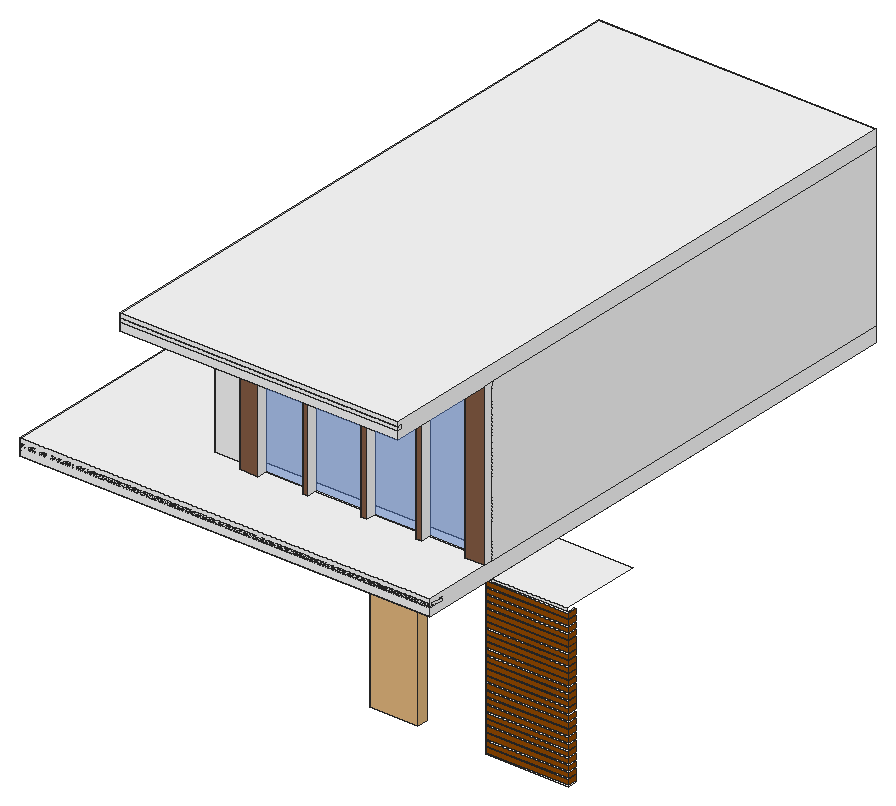
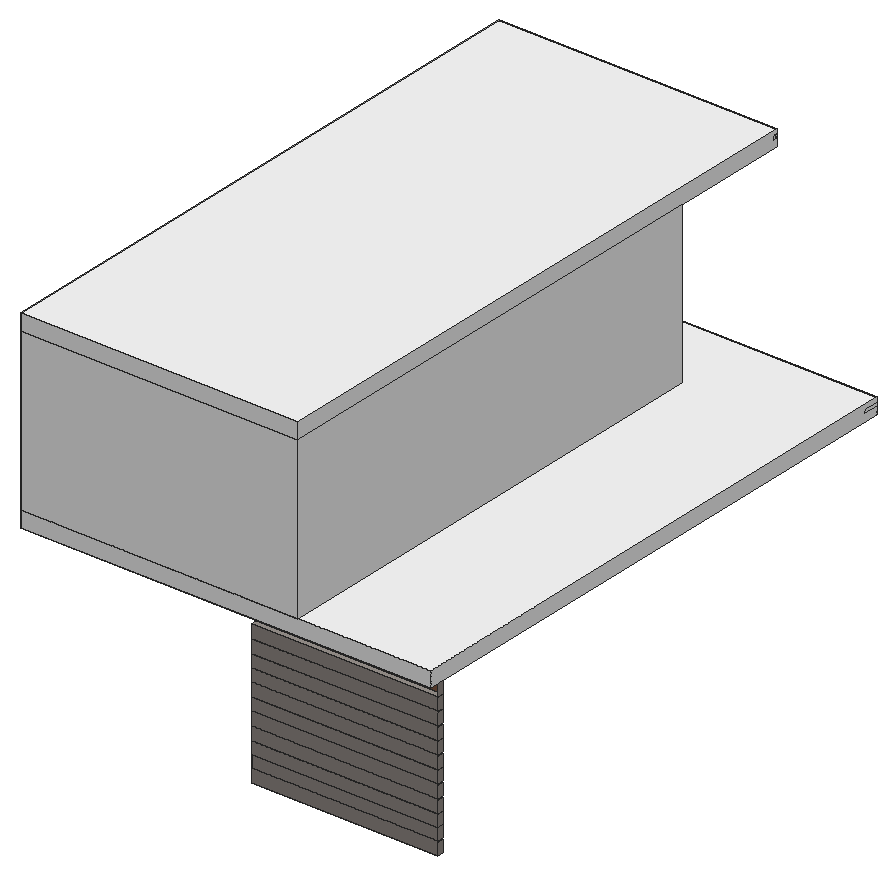
# SketchUp Ruby script. Lengths in inches.
U = 1.inch
M = Sketchup.active_model
def pt(a) = Geom::Point3d.new(a.map { |v| v * U })
def face(e, loops, mat)
  f = e.add_face(loops[0].map { |a| pt(a) })
  loops[1..].each { |l| e.add_face(l.map { |a| pt(a) }).erase! }
  f.material = f.back_material = mat if mat
  f
end
# faces: each face lists its corners as indices into pts; further lists are holes
def faces(e, pts, list, mat = nil) = list.each { |f| face(e, (f[0].is_a?(Array) ? f : [f]).map { |l| l.map { |i| pts[i] } }, mat) }
# xy, xz, yz: faces in a plane at the given z, y or x. An outline is a flat list of corners, or four numbers for a rectangle; further outlines are holes
def ring(l) = l.size == 4 ? [[l[0], l[1]], [l[2], l[1]], [l[2], l[3]], [l[0], l[3]]] : l.each_slice(2).to_a
def flat(e, list, mat, &to3) = list.each { |f| face(e, (f[0].is_a?(Array) ? f : [f]).map { |l| ring(l).map { |u, v| to3.(u, v) } }, mat) }
def xy(e, z, list, mat = nil) = flat(e, list, mat) { |x, y| [x, y, z] }
def xz(e, y, list, mat = nil) = flat(e, list, mat) { |x, z| [x, y, z] }
def yz(e, x, list, mat = nil) = flat(e, list, mat) { |y, z| [x, y, z] }
def lines(e, pts, list) = list.each { |a, b| e.add_line(pt(pts[a]), pt(pts[b])) }
# prism: a flat outline (further loops are holes) pulled along v
def prism(e, loops, v, mat = nil)
  f = face(e, loops, mat); d = Geom::Vector3d.new(v.map { |x| x * U })
  f.pushpull(f.normal.samedirection?(d) ? d.length : -d.length)
end
def box(e, o, s, mat = nil) = prism(e, [[o, [o[0] + s[0], o[1], o[2]], [o[0] + s[0], o[1] + s[1], o[2]], [o[0], o[1] + s[1], o[2]]]], [0, 0, s[2]], mat)
def at(x, y, z, deg = 0) = Geom::Transformation.translation(pt([x, y, z])) * Geom::Transformation.rotation(ORIGIN, Z_AXIS, deg.degrees)
def axes(o, x, y, z) = Geom::Transformation.new([*x, 0, *y, 0, *z, 0, *pt(o).to_a, 1])
def part(name) = M.definitions.add(name)
# library, detail: a bought-in or finely detailed component or shape, given as its bounding box
def library(name, o, s) = part(name).tap { |d| box(d.entities, o, s) }
def detail(e, o, s) = box(e.add_group.entities, o, s)
def put(e, d, t, mat = nil) = e.add_instance(d, t).tap { |i| i.material = mat if mat }
def group(e, t, mat = nil) = e.add_group.tap { |g| g.transformation = t; g.material = mat if mat }.entities
root = M.entities
M.materials.add("[Color C07]").color = [153, 76, 0]
M.materials.add("[Color M00]").color = [255, 255, 255]
M.materials.add("[Granite Tile]").color = [155, 148, 143]
M.materials.add("[Translucent Glass Blue]").color = [100, 149, 237]
M.materials["[Translucent Glass Blue]"].alpha = 0.5
M.materials.add("[Wood Veneer 02]").color = [137, 95, 70]
c1 = library("PINTU 6 YA",[0,-0.6875,0],[35.83,8.07,80.71])
box(root,[257.3125,155.5,390],[307.5,10.6875,2.42],"[Color M00]")
box(root,[356.51,125.125,522],[208.3,2.5625,3.02],"[Color M00]")
xy(root,265.59,[[561.375,211.8125,623.5625,211.8125,623.5625,218.625,622.25,218.625,622.25,213.625,561.375,213.625]],"[Color M00]")
xy(root,266.65,[[561.375,211.8125,561.375,213.625,622.25,213.625,622.25,218.625,623.5625,218.625,623.5625,211.8125]],"[Color M00]")
xy(root,268.5625,[[257.3125,562.2,396.75,566.64]],"[Granite Tile]")
xy(root,270.21,[[561.375,211.8125,623.5625,211.8125,623.5625,218.625,622.25,218.625,622.25,213.625,561.375,213.625]],"[Color M00]")
xy(root,271.27,[[561.375,211.8125,561.375,213.625,622.25,213.625,622.25,218.625,623.5625,218.625,623.5625,211.8125]],"[Color M00]")
xy(root,274.84,[[561.375,211.8125,623.5625,211.8125,623.5625,218.625,622.25,218.625,622.25,213.625,561.375,213.625]],"[Color M00]")
xy(root,276.02,[[561.375,211.8125,561.375,213.625,622.25,213.625,622.25,218.625,623.5625,218.625,623.5625,211.8125]],"[Color M00]")
xy(root,278.5,[[257.3125,562.2,396.75,566.64]],"[Granite Tile]")
xy(root,279.59,[[561.375,211.8125,623.5625,211.8125,623.5625,218.625,622.25,218.625,622.25,213.625,561.375,213.625]],"[Color M00]")
xy(root,280.85,[[561.375,211.8125,561.375,213.625,622.25,213.625,622.25,218.625,623.5625,218.625,623.5625,211.8125]],"[Color M00]")
xy(root,284.41,[[561.375,211.8125,623.5625,211.8125,623.5625,218.625,622.25,218.625,622.25,213.625,561.375,213.625]],"[Color M00]")
xy(root,285.72,[[561.375,211.8125,561.375,213.625,622.25,213.625,622.25,218.625,623.5625,218.625,623.5625,211.8125]],"[Color M00]")
xy(root,287.25,[[257.3125,562.2,396.75,566.64]],"[Granite Tile]")
xy(root,289.29,[[561.375,211.8125,623.5625,211.8125,623.5625,218.625,622.25,218.625,622.25,213.625,561.375,213.625]],"[Color M00]")
xy(root,290.1,[[561.375,211.8125,561.375,213.625,622.25,213.625,622.25,218.625,623.5625,218.625,623.5625,211.8125]],"[Color M00]")
xy(root,293.66,[[561.375,211.8125,623.5625,211.8125,623.5625,218.625,622.25,218.625,622.25,213.625,561.375,213.625]],"[Color M00]")
xy(root,294.97,[[561.375,211.8125,561.375,213.625,622.25,213.625,622.25,218.625,623.5625,218.625,623.5625,211.8125]],"[Color M00]")
xy(root,296.875,[[257.3125,562.2,396.75,566.64]],"[Granite Tile]")
xy(root,298.54,[[561.375,211.8125,623.5625,211.8125,623.5625,218.625,622.25,218.625,622.25,213.625,561.375,213.625]],"[Color M00]")
xy(root,299.91,[[561.375,211.8125,561.375,213.625,622.25,213.625,622.25,218.625,623.5625,218.625,623.5625,211.8125]],"[Color M00]")
xy(root,303.47,[[561.375,211.8125,623.5625,211.8125,623.5625,218.625,622.25,218.625,622.25,213.625,561.375,213.625]],"[Color M00]")
xy(root,304.72,[[561.375,211.8125,561.375,213.625,622.25,213.625,622.25,218.625,623.5625,218.625,623.5625,211.8125]],"[Color M00]")
xy(root,306.5,[[257.3125,562.2,396.75,566.64]],"[Granite Tile]")
xy(root,308.29,[[561.375,211.8125,623.5625,211.8125,623.5625,218.625,622.25,218.625,622.25,213.625,561.375,213.625]],"[Color M00]")
xy(root,309.6,[[561.375,211.8125,561.375,213.625,622.25,213.625,622.25,218.625,623.5625,218.625,623.5625,211.8125]],"[Color M00]")
xy(root,313.16,[[561.375,211.8125,623.5625,211.8125,623.5625,218.625,622.25,218.625,622.25,213.625,561.375,213.625]],"[Color M00]")
xy(root,314.54,[[561.375,211.8125,561.375,213.625,622.25,213.625,622.25,218.625,623.5625,218.625,623.5625,211.8125]],"[Color M00]")
xy(root,316.5625,[[257.3125,562.2,396.75,566.64]],"[Granite Tile]")
xy(root,318.1,[[561.375,211.8125,623.5625,211.8125,623.5625,218.625,622.25,218.625,622.25,213.625,561.375,213.625]],"[Color M00]")
xy(root,319.1,[[561.375,211.8125,561.375,213.625,622.25,213.625,622.25,218.625,623.5625,218.625,623.5625,211.8125]],"[Color M00]")
xy(root,322.66,[[561.375,211.8125,623.5625,211.8125,623.5625,218.625,622.25,218.625,622.25,213.625,561.375,213.625]],"[Color M00]")
xy(root,323.85,[[561.375,211.8125,561.375,213.625,622.25,213.625,622.25,218.625,623.5625,218.625,623.5625,211.8125]],"[Color M00]")
xy(root,326.4375,[[257.3125,562.2,396.75,566.64]],"[Granite Tile]")
xy(root,327.41,[[561.375,211.8125,623.5625,211.8125,623.5625,218.625,622.25,218.625,622.25,213.625,561.375,213.625]],"[Color M00]")
xy(root,328.35,[[561.375,211.8125,561.375,213.625,622.25,213.625,622.25,218.625,623.5625,218.625,623.5625,211.8125]],"[Color M00]")
xy(root,331.91,[[561.375,211.8125,623.5625,211.8125,623.5625,218.625,622.25,218.625,622.25,213.625,561.375,213.625]],"[Color M00]")
xy(root,333.1,[[561.375,211.8125,561.375,213.625,622.25,213.625,622.25,218.625,623.5625,218.625,623.5625,211.8125]],"[Color M00]")
xy(root,336.1875,[[257.3125,562.2,396.75,566.64]],"[Granite Tile]")
xy(root,336.66,[[561.375,211.8125,623.5625,211.8125,623.5625,218.625,622.25,218.625,622.25,213.625,561.375,213.625]],"[Color M00]")
xy(root,337.48,[[561.375,211.8125,561.375,213.625,622.25,213.625,622.25,218.625,623.5625,218.625,623.5625,211.8125]],"[Color M00]")
xy(root,341.04,[[561.375,211.8125,623.5625,211.8125,623.5625,218.625,622.25,218.625,622.25,213.625,561.375,213.625]],"[Color M00]")
xy(root,342.04,[[561.375,211.8125,561.375,213.625,622.25,213.625,622.25,218.625,623.5625,218.625,623.5625,211.8125]],"[Color M00]")
xy(root,345.6,[[561.375,211.8125,623.5625,211.8125,623.5625,218.625,622.25,218.625,622.25,213.625,561.375,213.625]],"[Color M00]")
xy(root,345.875,[[257.3125,562.2,396.75,566.64]],"[Granite Tile]")
xy(root,346.54,[[561.375,211.8125,561.375,213.625,622.25,213.625,622.25,218.625,623.5625,218.625,623.5625,211.8125]],"[Color M00]")
xy(root,350.1,[[561.375,211.8125,623.5625,211.8125,623.5625,218.625,622.25,218.625,622.25,213.625,561.375,213.625]],"[Color M00]")
xy(root,350.85,[[561.375,211.8125,561.375,213.625,622.25,213.625,622.25,218.625,623.5625,218.625,623.5625,211.8125]],"[Color M00]")
xy(root,354.41,[[561.375,211.8125,623.5625,211.8125,623.5625,218.625,622.25,218.625,622.25,213.625,561.375,213.625]],"[Color M00]")
xy(root,355.35,[[561.375,211.8125,561.375,213.625,622.25,213.625,622.25,218.625,623.5625,218.625,623.5625,211.8125]],"[Color M00]")
xy(root,355.4375,[[257.3125,562.2,396.75,566.64]],"[Granite Tile]")
xy(root,358.91,[[561.375,211.8125,623.5625,211.8125,623.5625,218.625,622.25,218.625,622.25,213.625,561.375,213.625]],"[Color M00]")
xy(root,359.73,[[561.375,211.8125,561.375,213.625,622.25,213.625,622.25,218.625,623.5625,218.625,623.5625,211.8125]],"[Color M00]")
xy(root,363.29,[[561.375,211.8125,623.5625,211.8125,623.5625,218.625,622.25,218.625,622.25,213.625,561.375,213.625]],"[Color M00]")
xy(root,364.29,[[561.375,211.8125,561.375,213.625,622.25,213.625,622.25,218.625,623.5625,218.625,623.5625,211.8125]],"[Color M00]")
xy(root,365.5,[[257.3125,562.2,396.75,566.64]],"[Granite Tile]")
xy(root,367.85,[[561.375,211.8125,623.5625,211.8125,623.5625,218.625,622.25,218.625,622.25,213.625,561.375,213.625]],"[Color M00]")
xy(root,368.98,[[561.375,211.8125,561.375,213.625,622.25,213.625,622.25,218.625,623.5625,218.625,623.5625,211.8125]],"[Color M00]")
xy(root,372.54,[[561.375,211.8125,623.5625,211.8125,623.5625,218.625,622.25,218.625,622.25,213.625,561.375,213.625]],"[Color M00]")
xy(root,373.79,[[561.375,211.8125,561.375,213.625,622.25,213.625,622.25,218.625,623.5625,218.625,623.5625,211.8125]],"[Color M00]")
xy(root,375.25,[[257.3125,562.2,396.75,566.64]],"[Granite Tile]")
xy(root,377.35,[[561.375,211.8125,623.5625,211.8125,623.5625,218.625,622.25,218.625,622.25,213.625,561.375,213.625]],"[Color M00]")
xy(root,378.41,[[561.375,211.8125,561.375,213.625,622.25,213.625,622.25,218.625,623.5625,218.625,623.5625,211.8125]],"[Color M00]")
xy(root,381.98,[[561.375,211.8125,623.5625,211.8125,623.5625,218.625,622.25,218.625,622.25,213.625,561.375,213.625]],"[Color M00]")
xy(root,384,[[[396.75,213.625,564.8125,573.625],[405.75,222.625,555.8125,564.625]],[564.8125,213.625,620.9375,275.23]],"[Color M00]")
xy(root,384,[[257.3125,562.2,396.75,573.625]],"[Granite Tile]")
xy(root,396,[[[381.19,206.5,381.19,213.625,356.51,213.625,356.51,573.625,564.8125,573.625,564.8125,213.625,395.01,213.625,395.01,206.5],[365.51,222.625,555.8125,564.625]],[428.46,206.5,432.18,213.625],[472.11,206.5,476.51,213.625],[513.36,206.5,517.77,213.625],[550.21,206.5,564.8125,213.625],
  [365.51,222.625,555.8125,564.625]],"[Color M00]")
xy(root,502.09,[[395.01,206.5,428.46,213.625],[432.18,206.5,472.11,213.625],[476.51,206.5,513.36,213.625],[517.77,206.5,550.21,213.625]],"[Color M00]")
xy(root,516,[[381.19,206.5,564.8125,213.625],[[356.51,213.625,564.8125,573.625],[365.51,222.625,555.8125,564.625]]],"[Color M00]")
xz(root,206.5,[[381.19,396,395.01,396,395.01,502.09,428.46,502.09,428.46,396,432.18,396,432.18,502.09,472.11,502.09,472.11,396,476.51,396,476.51,502.09,513.36,502.09,513.36,396,517.77,396,517.77,502.09,550.21,502.09,550.21,396,564.8125,396,564.8125,516,381.19,516]],"[Wood Veneer 02]")
xz(root,211.8125,[[561.375,266.65,623.5625,270.21],[561.375,271.27,623.5625,274.84],[561.375,276.02,623.5625,279.59],[561.375,280.85,623.5625,284.41],[561.375,285.72,623.5625,289.29],
  [561.375,290.1,623.5625,293.66],[561.375,294.97,623.5625,298.54],[561.375,299.91,623.5625,303.47],[561.375,304.72,623.5625,308.29],[561.375,309.6,623.5625,313.16],
  [561.375,314.54,623.5625,318.1],[561.375,319.1,623.5625,322.66],[561.375,323.85,623.5625,327.41],[561.375,328.35,623.5625,331.91],[561.375,333.1,623.5625,336.66],
  [561.375,337.48,623.5625,341.04],[561.375,342.04,623.5625,345.6],[561.375,346.54,623.5625,350.1],[561.375,350.85,623.5625,354.41],[561.375,355.35,623.5625,358.91],
  [561.375,359.73,623.5625,363.29],[561.375,364.29,623.5625,367.85],[561.375,368.98,623.5625,372.54],[561.375,373.79,623.5625,377.35],[561.375,378.41,623.5625,381.98]],"[Color C07]")
xz(root,213.625,[[561.375,266.65,564.8125,270.21],[561.375,271.27,564.8125,274.84],[561.375,276.02,564.8125,279.59],[561.375,280.85,564.8125,284.41],[561.375,285.72,564.8125,289.29],
  [561.375,290.1,564.8125,293.66],[561.375,294.97,564.8125,298.54],[561.375,299.91,564.8125,303.47],[561.375,304.72,564.8125,308.29],[561.375,309.6,564.8125,313.16],
  [561.375,314.54,564.8125,318.1],[561.375,319.1,564.8125,322.66],[561.375,323.85,564.8125,327.41],[561.375,328.35,564.8125,331.91],[561.375,333.1,564.8125,336.66],
  [561.375,337.48,564.8125,341.04],[561.375,342.04,564.8125,345.6],[561.375,346.54,564.8125,350.1],[561.375,350.85,564.8125,354.41],[561.375,355.35,564.8125,358.91],
  [561.375,359.73,564.8125,363.29],[561.375,364.29,564.8125,367.85],[561.375,368.98,564.8125,372.54],[561.375,373.79,564.8125,377.35],[561.375,378.41,564.8125,381.98],
  [620.9375,378.41,622.25,381.98],[564.8125,381.98,620.9375,384],[356.51,396,381.19,516]],"[Color M00]")
xz(root,213.625,[[564.8125,265.59,620.9375,266.65],[564.8125,266.65,620.9375,270.21],[564.8125,270.21,620.9375,271.27],[564.8125,271.27,620.9375,274.84],[564.8125,274.84,620.9375,276.02],
  [564.8125,276.02,620.9375,279.59],[564.8125,279.59,620.9375,280.85],[564.8125,280.85,620.9375,284.41],[564.8125,284.41,620.9375,285.72],[564.8125,285.72,620.9375,289.29],
  [564.8125,289.29,620.9375,290.1],[564.8125,290.1,620.9375,293.66],[564.8125,293.66,620.9375,294.97],[564.8125,294.97,620.9375,298.54],[564.8125,298.54,620.9375,299.91],
  [564.8125,299.91,620.9375,303.47],[564.8125,303.47,620.9375,304.72],[564.8125,304.72,620.9375,308.29],[564.8125,308.29,620.9375,309.6],[564.8125,309.6,620.9375,313.16],
  [564.8125,313.16,620.9375,314.54],[564.8125,314.54,620.9375,318.1],[564.8125,318.1,620.9375,319.1],[564.8125,319.1,620.9375,322.66],[564.8125,322.66,620.9375,323.85],
  [564.8125,323.85,620.9375,327.41],[564.8125,327.41,620.9375,328.35],[564.8125,328.35,620.9375,331.91],[564.8125,331.91,620.9375,333.1],[564.8125,333.1,620.9375,336.66],
  [564.8125,336.66,620.9375,337.48],[564.8125,337.48,620.9375,341.04],[564.8125,341.04,620.9375,342.04],[564.8125,342.04,620.9375,345.6],[564.8125,345.6,620.9375,346.54],
  [564.8125,346.54,620.9375,350.1],[564.8125,350.1,620.9375,350.85],[564.8125,350.85,620.9375,354.41],[564.8125,354.41,620.9375,355.35],[564.8125,355.35,620.9375,358.91],
  [564.8125,358.91,620.9375,359.73],[564.8125,359.73,620.9375,363.29],[564.8125,363.29,620.9375,364.29],[564.8125,364.29,620.9375,367.85],[564.8125,367.85,620.9375,368.98],
  [564.8125,368.98,620.9375,372.54],[564.8125,372.54,620.9375,373.79],[564.8125,373.79,620.9375,377.35],[564.8125,377.35,620.9375,378.41],[395.01,396,428.46,502.09],
  [432.18,396,472.11,502.09],[476.51,396,513.36,502.09],[517.77,396,550.21,502.09]],"[Translucent Glass Blue]")
xz(root,218.625,[[622.25,266.65,623.5625,270.21],[622.25,271.27,623.5625,274.84],[622.25,276.02,623.5625,279.59],[622.25,280.85,623.5625,284.41],[622.25,285.72,623.5625,289.29],
  [622.25,290.1,623.5625,293.66],[622.25,294.97,623.5625,298.54],[622.25,299.91,623.5625,303.47],[622.25,304.72,623.5625,308.29],[622.25,309.6,623.5625,313.16],
  [622.25,314.54,623.5625,318.1],[622.25,319.1,623.5625,322.66],[622.25,323.85,623.5625,327.41],[622.25,328.35,623.5625,331.91],[622.25,333.1,623.5625,336.66],
  [622.25,337.48,623.5625,341.04],[622.25,342.04,623.5625,345.6],[622.25,346.54,623.5625,350.1],[622.25,350.85,623.5625,354.41],[622.25,355.35,623.5625,358.91],
  [622.25,359.73,623.5625,363.29],[622.25,364.29,623.5625,367.85],[622.25,368.98,623.5625,372.54],[622.25,373.79,623.5625,377.35],[622.25,378.41,623.5625,381.98]],"[Color M00]")
xz(root,222.625,[[365.51,396,555.8125,516]],"[Color M00]")
xz(root,562.2,[[257.3125,268.5625,396.75,277.3125],[257.3125,278.5,396.75,287.25],[257.3125,287.25,396.75,296],[257.3125,296.875,396.75,305.625],[257.3125,306.5,396.75,315.25],
  [257.3125,316.5625,396.75,325.3125],[257.3125,326.4375,396.75,335.1875],[257.3125,336.1875,396.75,344.9375],[257.3125,345.875,396.75,354.625],[257.3125,355.4375,396.75,364.1875],
  [257.3125,365.5,396.75,374.25],[257.3125,375.25,396.75,384]],"[Wood Veneer 02]")
xz(root,564.625,[[365.51,396,555.8125,516]],"[Color M00]")
xz(root,566.64,[[257.3125,268.5625,396.75,278.5],[257.3125,278.5,396.75,287.25],[257.3125,287.25,396.75,296.875],[257.3125,296.875,396.75,306.5],[257.3125,306.5,396.75,316.5625],
  [257.3125,316.5625,396.75,326.4375],[257.3125,326.4375,396.75,336.1875],[257.3125,336.1875,396.75,345.875],[257.3125,345.875,396.75,355.4375],[257.3125,355.4375,396.75,365.5],
  [257.3125,365.5,396.75,375.25]],"[Granite Tile]")
xz(root,573.625,[[356.51,396,564.8125,516]],"[Color M00]")
yz(root,257.3125,[[562.2,268.5625,566.64,277.3125],[562.2,278.5,566.64,287.25],[562.2,287.25,566.64,296],[562.2,296.875,566.64,305.625],[562.2,306.5,566.64,315.25],
  [562.2,316.5625,566.64,325.3125],[562.2,326.4375,566.64,335.1875],[562.2,336.1875,566.64,344.9375],[562.2,345.875,566.64,354.625],[562.2,355.4375,566.64,364.1875],
  [562.2,365.5,566.64,374.25],[562.2,375.25,566.64,384]],"[Granite Tile]")
yz(root,356.51,[[213.625,396,573.625,516]],"[Color M00]")
yz(root,365.51,[[222.625,396,564.625,516]],"[Color M00]")
yz(root,381.19,[[206.5,396,213.625,516]],"[Color M00]")
yz(root,395.01,[[206.5,396,213.625,502.09]],"[Color M00]")
yz(root,396.75,[[562.2,278.5,566.64,287.25]],"[Color M00]")
yz(root,428.46,[[206.5,396,213.625,502.09]],"[Color M00]")
yz(root,432.18,[[206.5,396,213.625,502.09]],"[Color M00]")
yz(root,472.11,[[206.5,396,213.625,502.09]],"[Color M00]")
yz(root,476.51,[[206.5,396,213.625,502.09]],"[Color M00]")
yz(root,513.36,[[206.5,396,213.625,502.09]],"[Color M00]")
yz(root,517.77,[[206.5,396,213.625,502.09]],"[Color M00]")
yz(root,550.21,[[206.5,396,213.625,502.09]],"[Color M00]")
yz(root,555.8125,[[222.625,396,564.625,516]],"[Color M00]")
yz(root,561.375,[[211.8125,266.65,213.625,270.21],[211.8125,271.27,213.625,274.84],[211.8125,276.02,213.625,279.59],[211.8125,280.85,213.625,284.41],[211.8125,285.72,213.625,289.29],
  [211.8125,290.1,213.625,293.66],[211.8125,294.97,213.625,298.54],[211.8125,299.91,213.625,303.47],[211.8125,304.72,213.625,308.29],[211.8125,309.6,213.625,313.16],
  [211.8125,314.54,213.625,318.1],[211.8125,319.1,213.625,322.66],[211.8125,323.85,213.625,327.41],[211.8125,328.35,213.625,331.91],[211.8125,333.1,213.625,336.66],
  [211.8125,337.48,213.625,341.04],[211.8125,342.04,213.625,345.6],[211.8125,346.54,213.625,350.1],[211.8125,350.85,213.625,354.41],[211.8125,355.35,213.625,358.91],
  [211.8125,359.73,213.625,363.29],[211.8125,364.29,213.625,367.85],[211.8125,368.98,213.625,372.54],[211.8125,373.79,213.625,377.35],[211.8125,378.41,213.625,381.98]],"[Color M00]")
yz(root,564.8125,[[206.5,396,213.625,516],[213.625,396,573.625,516]],"[Color M00]")
yz(root,622.25,[[213.625,378.41,218.625,381.98]],"[Color M00]")
yz(root,623.5625,[[211.8125,266.65,218.625,270.21],[211.8125,271.27,218.625,274.84],[211.8125,276.02,218.625,279.59],[211.8125,280.85,218.625,284.41],[211.8125,285.72,218.625,289.29],
  [211.8125,290.1,218.625,293.66],[211.8125,294.97,218.625,298.54],[211.8125,299.91,218.625,303.47],[211.8125,304.72,218.625,308.29],[211.8125,309.6,218.625,313.16],
  [211.8125,314.54,218.625,318.1],[211.8125,319.1,218.625,322.66],[211.8125,323.85,218.625,327.41],[211.8125,328.35,218.625,331.91],[211.8125,333.1,218.625,336.66],
  [211.8125,337.48,218.625,341.04],[211.8125,342.04,218.625,345.6],[211.8125,346.54,218.625,350.1],[211.8125,350.85,218.625,354.41],[211.8125,355.35,218.625,358.91],
  [211.8125,359.73,218.625,363.29],[211.8125,364.29,218.625,367.85],[211.8125,368.98,218.625,372.54],[211.8125,373.79,218.625,377.35],[211.8125,378.41,218.625,381.98]],"[Color C07]")
put(root,c1,at(479.58,206.24,271.25),"[Granite Tile]")
g1 = group(root,at(396.75,573.625,384),"[Color M00]")
box(g1,[-139.4375,-418.125,0],[307.5,418.125,12])
g2 = group(root,at(356.51,573.625,516),"[Color M00]")
box(g2,[0,-448.5,0],[208.3,448.5,12])
